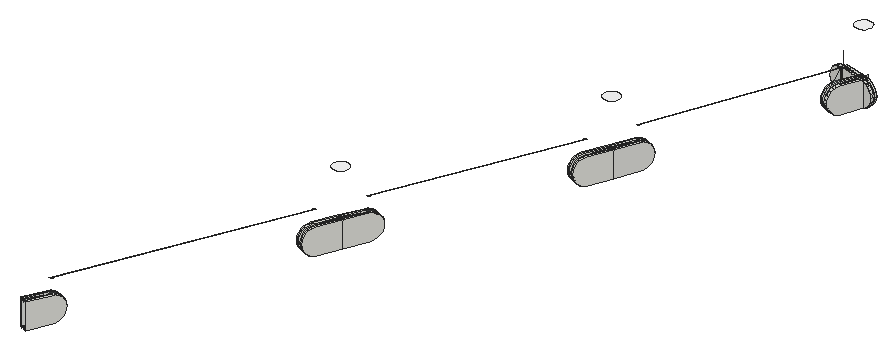
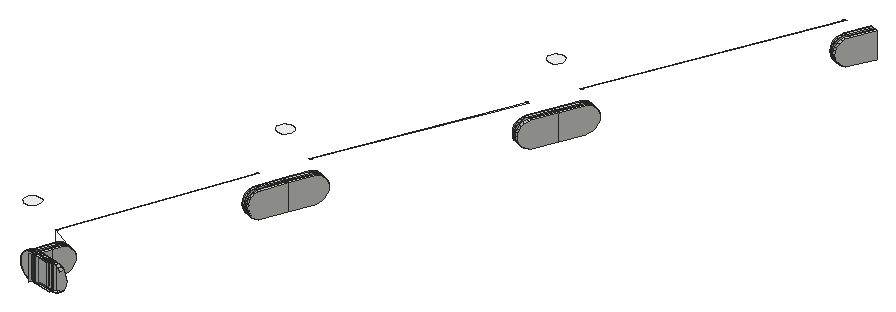
# SketchUp Ruby script. Lengths in inches.
U = 1.inch
M = Sketchup.active_model
def pt(a) = Geom::Point3d.new(a.map { |v| v * U })
def face(e, loops, mat)
  f = e.add_face(loops[0].map { |a| pt(a) })
  loops[1..].each { |l| e.add_face(l.map { |a| pt(a) }).erase! }
  f.material = f.back_material = mat if mat
  f
end
# faces: each face lists its corners as indices into pts; further lists are holes
def faces(e, pts, list, mat = nil) = list.each { |f| face(e, (f[0].is_a?(Array) ? f : [f]).map { |l| l.map { |i| pts[i] } }, mat) }
# xy, xz, yz: faces in a plane at the given z, y or x. An outline is a flat list of corners, or four numbers for a rectangle; further outlines are holes
def ring(l) = l.size == 4 ? [[l[0], l[1]], [l[2], l[1]], [l[2], l[3]], [l[0], l[3]]] : l.each_slice(2).to_a
def flat(e, list, mat, &to3) = list.each { |f| face(e, (f[0].is_a?(Array) ? f : [f]).map { |l| ring(l).map { |u, v| to3.(u, v) } }, mat) }
def xy(e, z, list, mat = nil) = flat(e, list, mat) { |x, y| [x, y, z] }
def xz(e, y, list, mat = nil) = flat(e, list, mat) { |x, z| [x, y, z] }
def yz(e, x, list, mat = nil) = flat(e, list, mat) { |y, z| [x, y, z] }
def lines(e, pts, list) = list.each { |a, b| e.add_line(pt(pts[a]), pt(pts[b])) }
# prism: a flat outline (further loops are holes) pulled along v
def prism(e, loops, v, mat = nil)
  f = face(e, loops, mat); d = Geom::Vector3d.new(v.map { |x| x * U })
  f.pushpull(f.normal.samedirection?(d) ? d.length : -d.length)
end
def box(e, o, s, mat = nil) = prism(e, [[o, [o[0] + s[0], o[1], o[2]], [o[0] + s[0], o[1] + s[1], o[2]], [o[0], o[1] + s[1], o[2]]]], [0, 0, s[2]], mat)
def at(x, y, z, deg = 0) = Geom::Transformation.translation(pt([x, y, z])) * Geom::Transformation.rotation(ORIGIN, Z_AXIS, deg.degrees)
def axes(o, x, y, z) = Geom::Transformation.new([*x, 0, *y, 0, *z, 0, *pt(o).to_a, 1])
def part(name) = M.definitions.add(name)
# library, detail: a bought-in or finely detailed component or shape, given as its bounding box
def library(name, o, s) = part(name).tap { |d| box(d.entities, o, s) }
def detail(e, o, s) = box(e.add_group.entities, o, s)
def put(e, d, t, mat = nil) = e.add_instance(d, t).tap { |i| i.material = mat if mat }
def group(e, t, mat = nil) = e.add_group.tap { |g| g.transformation = t; g.material = mat if mat }.entities
root = M.entities
M.materials.add("Glass_Safety_01").color = [204, 235, 244]
M.materials["Glass_Safety_01"].alpha = 0.1
M.materials.add("[Color_000]").color = [255, 255, 255]
xy(root,351.283,[[999.992,955.024,999.739,955.134,1000.525,956.939,1000.778,956.828],[999.558,955.212,999.306,955.322,1000.092,957.127,1000.344,957.017],[1008.551,974.677,1008.298,974.787,1008.365,974.939,1009.084,976.592,1009.337,976.482],[1008.118,974.865,1007.865,974.976,1008.651,976.78,1008.904,976.67,1008.184,975.017],[1009.337,976.482,1009.084,976.592,1009.871,978.396,1010.123,978.286],
  [1008.904,976.67,1008.651,976.78,1009.4375,978.585,1009.69,978.475],[1016.523,992.981,1016.271,993.091,1016.348,993.269,1017.057,994.896,1017.309,994.786],[1016.09,993.17,1015.837,993.28,1016.618,995.072,1016.875,994.971,1016.168,993.348],[1017.315,994.799,1017.058,994.9,1017.774,996.733,1018.031,996.633],[1016.875,994.971,1016.618,995.072,1016.621,995.078,1016.624,995.085,1016.876,994.975],
  [1016.876,994.975,1016.624,995.085,1017.334,996.905,1017.591,996.805],[1023.511,1010.674,1023.255,1010.774,1023.329,1010.964,1023.838,1012.27,1023.906,1012.255,1023.948,1012.447,1023.965,1012.524,1023.982,1012.603,1024.227,1012.508],[1023.071,1010.846,1022.815,1010.946,1023.371,1012.372,1023.644,1012.3125,1023.145,1011.036],[1023.906,1012.255,1023.838,1012.27,1023.911,1012.456,1023.948,1012.447],[1023.838,1012.27,1023.799,1012.279,1023.841,1012.471,1023.911,1012.456],
  [1023.799,1012.279,1023.644,1012.3125,1023.716,1012.498,1023.841,1012.471],[1023.644,1012.3125,1023.371,1012.372,1023.444,1012.558,1023.716,1012.498],[1023.371,1012.372,1021.983,1012.675,1022.025,1012.868,1023.251,1012.599,1023.444,1012.558],[1023.948,1012.447,1023.911,1012.456,1023.94,1012.53,1023.965,1012.524],[1023.911,1012.456,1023.841,1012.471,1023.858,1012.548,1023.94,1012.53],
  [1023.841,1012.471,1023.716,1012.498,1023.745,1012.572,1023.858,1012.548],[1023.716,1012.498,1023.444,1012.558,1023.473,1012.632,1023.745,1012.572],[1023.965,1012.524,1023.94,1012.53,1023.97,1012.608,1023.982,1012.603],[1023.94,1012.53,1023.858,1012.548,1023.745,1012.572,1023.787,1012.68,1023.53,1012.78,1023.473,1012.632,1022.042,1012.945,1022.084,1013.137,1022.095,1013.134,1022.105,1013.13,1022.106,1013.132,1023.9,1012.74,1024.007,1012.717,1023.982,1012.603,1023.97,1012.608],[1023.444,1012.558,1023.251,1012.599,1022.025,1012.868,1022.042,1012.945,1023.473,1012.632],
  [1023.745,1012.572,1023.473,1012.632,1023.53,1012.78,1023.787,1012.68],[1021.983,1012.675,1021.876,1012.699,1021.879,1012.714,1021.903,1012.702,1022.02,1012.949,1022.042,1012.945,1022.025,1012.868],[1021.903,1012.702,1021.879,1012.714,1021.935,1012.968,1022.02,1012.949]])
xy(root,351.362,[[1008.456,975.148,1008.275,975.226,1008.904,976.67,1009.084,976.592],[1009.084,976.592,1008.904,976.67,1009.533,978.114,1009.713,978.035],[1016.428,993.452,1016.247,993.531,1016.875,994.971,1016.966,994.936,1017.057,994.896],[1017.058,994.9,1016.966,994.936,1016.876,994.975,1017.447,996.438,1017.631,996.367],[1016.966,994.936,1016.875,994.971,1016.875,994.973,1016.876,994.975],
  [1023.398,1011.141,1023.214,1011.213,1023.745,1012.572,1023.858,1012.548,1023.879,1012.644,1023.97,1012.608],[1023.858,1012.548,1023.745,1012.572,1023.787,1012.68,1023.879,1012.644],[1023.745,1012.572,1023.58,1012.608,1023.622,1012.801,1023.9,1012.74,1023.879,1012.644,1023.787,1012.68],[1023.58,1012.608,1022.319,1012.884,1022.361,1013.076,1023.622,1012.801]],"Glass_Safety_01")
xy(root,353.33,[[999.739,955.134,1000.368,956.578,1000.187,956.656,999.558,955.212],[1008.456,975.148,1009.084,976.592,1008.904,976.67,1008.275,975.226],[1009.084,976.592,1009.713,978.035,1009.533,978.114,1008.904,976.67],[1016.428,993.452,1017.057,994.896,1016.966,994.936,1016.875,994.971,1016.247,993.531],[1017.058,994.9,1017.631,996.367,1017.447,996.438,1016.876,994.975,1016.966,994.936],
  [1016.966,994.936,1016.876,994.975,1016.875,994.973,1016.875,994.971],[1023.398,1011.141,1023.97,1012.608,1023.879,1012.644,1023.858,1012.548,1023.745,1012.572,1023.214,1011.213],[1023.858,1012.548,1023.879,1012.644,1023.787,1012.68,1023.745,1012.572],[1023.745,1012.572,1023.787,1012.68,1023.879,1012.644,1023.9,1012.74,1023.622,1012.801,1023.58,1012.608],[1023.58,1012.608,1023.622,1012.801,1022.361,1013.076,1022.319,1012.884]],"Glass_Safety_01")
xy(root,353.409,[[999.992,955.024,1000.778,956.828,1000.525,956.939,999.739,955.134],[999.558,955.212,1000.344,957.017,1000.092,957.127,999.306,955.322],[1008.551,974.677,1009.337,976.482,1009.084,976.592,1008.365,974.939,1008.298,974.787],[1008.118,974.865,1008.184,975.017,1008.904,976.67,1008.651,976.78,1007.865,974.976],[1009.337,976.482,1010.123,978.286,1009.871,978.396,1009.084,976.592],
  [1008.904,976.67,1009.69,978.475,1009.4375,978.585,1008.651,976.78],[1016.523,992.981,1017.309,994.786,1017.057,994.896,1016.348,993.269,1016.271,993.091],[1016.09,993.17,1016.168,993.348,1016.875,994.971,1016.618,995.072,1015.837,993.28],[1017.315,994.799,1018.031,996.633,1017.774,996.733,1017.058,994.9],[1016.875,994.971,1016.876,994.975,1016.624,995.085,1016.621,995.078,1016.618,995.072],
  [1016.876,994.975,1017.591,996.805,1017.334,996.905,1016.624,995.085],[1023.511,1010.674,1024.227,1012.508,1023.982,1012.603,1023.965,1012.524,1023.948,1012.447,1023.906,1012.255,1023.838,1012.27,1023.329,1010.964,1023.255,1010.774],[1023.071,1010.846,1023.145,1011.036,1023.644,1012.3125,1023.371,1012.372,1022.815,1010.946],[1023.906,1012.255,1023.948,1012.447,1023.911,1012.456,1023.838,1012.27],[1023.838,1012.27,1023.911,1012.456,1023.841,1012.471,1023.799,1012.279],
  [1023.799,1012.279,1023.841,1012.471,1023.716,1012.498,1023.644,1012.3125],[1023.644,1012.3125,1023.716,1012.498,1023.444,1012.558,1023.371,1012.372],[1023.371,1012.372,1023.444,1012.558,1023.251,1012.599,1022.025,1012.868,1021.983,1012.675],[1023.948,1012.447,1023.965,1012.524,1023.94,1012.53,1023.911,1012.456],[1023.911,1012.456,1023.94,1012.53,1023.858,1012.548,1023.841,1012.471],
  [1023.841,1012.471,1023.858,1012.548,1023.745,1012.572,1023.716,1012.498],[1023.716,1012.498,1023.745,1012.572,1023.473,1012.632,1023.444,1012.558],[1023.965,1012.524,1023.982,1012.603,1023.97,1012.608,1023.94,1012.53],[1023.94,1012.53,1023.97,1012.608,1023.982,1012.603,1024.007,1012.717,1023.9,1012.74,1022.106,1013.132,1022.105,1013.13,1022.095,1013.134,1022.084,1013.137,1022.042,1012.945,1023.473,1012.632,1023.53,1012.78,1023.787,1012.68,1023.745,1012.572,1023.858,1012.548],[1023.444,1012.558,1023.473,1012.632,1022.042,1012.945,1022.025,1012.868,1023.251,1012.599],
  [1023.745,1012.572,1023.787,1012.68,1023.53,1012.78,1023.473,1012.632],[1021.983,1012.675,1022.025,1012.868,1022.042,1012.945,1022.02,1012.949,1021.903,1012.702,1021.879,1012.714,1021.876,1012.699],[1021.903,1012.702,1022.02,1012.949,1021.935,1012.968,1021.879,1012.714]])
xy(root,354.511,[[1000.525,956.939,1008.184,975.017,1000.344,957.017],[1000.525,956.939,1008.365,974.939,1008.184,975.017],[1009.871,978.396,1016.168,993.348,1009.69,978.475],[1009.871,978.396,1016.348,993.269,1016.168,993.348],[1017.774,996.733,1023.145,1011.036,1017.591,996.805],
  [1017.774,996.733,1023.329,1010.964,1023.145,1011.036]],"Glass_Safety_01")
xy(root,357.267,[[1009.039,976.003,1009.2,976.036,1009.347,976.109,1009.47,976.219,1009.561,976.356,1009.613,976.512,1009.623,976.676,1009.589,976.837,1009.516,976.984,1009.407,977.107,1009.269,977.198,1009.113,977.25,1008.949,977.259,1008.788,977.226,1008.641,977.153,1008.518,977.043,1008.428,976.906,1008.376,976.75,1008.366,976.586,1008.399,976.425,1008.473,976.278,1008.582,976.155,1008.719,976.064,1008.875,976.012],[1017.011,994.307,1017.173,994.34,1017.32,994.414,1017.443,994.523,1017.533,994.66,1017.585,994.816,1017.595,994.981,1017.562,995.142,1017.488,995.289,1017.379,995.412,1017.242,995.502,1017.086,995.554,1016.921,995.564,1016.76,995.531,1016.613,995.457,1016.49,995.348,1016.4,995.211,1016.348,995.055,1016.338,994.89,1016.371,994.729,1016.445,994.582,1016.554,994.459,1016.691,994.369,1016.847,994.317],[1023.924,1012.016,1024.085,1012.049,1024.232,1012.122,1024.355,1012.231,1024.445,1012.369,1024.497,1012.525,1024.507,1012.689,1024.474,1012.85,1024.4,1012.997,1024.291,1013.12,1024.154,1013.211,1023.998,1013.262,1023.834,1013.272,1023.673,1013.239,1023.526,1013.166,1023.403,1013.056,1023.312,1012.919,1023.26,1012.763,1023.25,1012.599,1023.284,1012.438,1023.357,1012.291,1023.466,1012.168,1023.604,1012.077,1023.76,1012.025]],"[Color_000]")
p = [[1000.778,956.828,353.409],[999.992,955.024,353.409],[999.992,955.024,351.283],[1000.778,956.828,351.283],[1000.887,957.081,351.319],[1000.99,957.316,351.425],
  [1001.078,957.518,351.594],[1001.145,957.672,351.814],[1001.1875,957.77,352.071],[1001.202,957.803,352.346],[1001.1875,957.77,352.621],[1001.145,957.672,352.877],
  [1001.078,957.518,353.098],[1000.99,957.316,353.267],[1000.887,957.081,353.373],[999.739,955.134,353.409],[1000.525,956.939,353.409],[1000.525,956.939,351.283],
  [999.739,955.134,351.283],[999.739,955.134,351.362],[1000.368,956.578,351.362],[1000.368,956.578,353.33],[999.739,955.134,353.33],[999.558,955.212,351.283],
  [1000.344,957.017,351.283],[1000.344,957.017,353.409],[999.558,955.212,353.409],[999.558,955.212,353.33],[1000.187,956.656,353.33],[1000.187,956.656,351.362],
  [999.558,955.212,351.362],[999.306,955.322,353.409],[1000.092,957.127,353.409],[1000.202,957.379,353.373],[1000.304,957.614,353.267],[1000.392,957.816,353.098],
  [1000.459,957.971,352.877],[1000.502,958.069,352.621],[1000.516,958.102,352.346],[1000.502,958.069,352.071],[1000.459,957.971,351.814],[1000.392,957.816,351.594],
  [1000.304,957.614,351.425],[1000.202,957.379,351.319],[1000.092,957.127,351.283],[999.306,955.322,351.283],[1000.635,957.191,351.319],[1000.737,957.426,351.425],
  [1000.825,957.628,351.594],[1000.893,957.783,351.814],[1000.935,957.88,352.071],[1000.949,957.913,352.346],[1000.935,957.88,352.621],[1000.893,957.783,352.877],
  [1000.825,957.628,353.098],[1000.737,957.426,353.267],[1000.635,957.191,353.373],[1000.454,957.269,351.319],[1000.454,957.269,353.373],[1000.557,957.504,353.267],
  [1000.645,957.706,353.098],[1000.712,957.861,352.877],[1000.754,957.958,352.621],[1000.769,957.992,352.346],[1000.754,957.958,352.071],[1000.712,957.861,351.814],
  [1000.645,957.706,351.594],[1000.557,957.504,351.425],[1009.337,976.482,353.409],[1008.551,974.677,353.409],[1008.441,974.425,353.373],[1008.339,974.19,353.267],
  [1008.251,973.988,353.098],[1008.184,973.833,352.877],[1008.141,973.735,352.621],[1008.127,973.702,352.346],[1008.141,973.735,352.071],[1008.184,973.833,351.814],
  [1008.251,973.988,351.594],[1008.339,974.19,351.425],[1008.441,974.425,351.319],[1008.551,974.677,351.283],[1009.337,976.482,351.283],[1008.298,974.787,353.409],
  [1008.365,974.939,353.409],[1008.365,974.939,351.283],[1008.298,974.787,351.283],[1008.189,974.535,351.319],[1008.086,974.3,351.425],[1007.998,974.098,351.594],
  [1007.931,973.943,351.814],[1007.888,973.846,352.071],[1007.874,973.8125,352.346],[1007.888,973.846,352.621],[1007.931,973.943,352.877],[1007.998,974.098,353.098],
  [1008.086,974.3,353.267],[1008.189,974.535,353.373],[1008.118,974.865,351.283],[1008.184,975.017,351.283],[1008.184,975.017,353.409],[1008.118,974.865,353.409],
  [1008.008,974.613,353.373],[1007.906,974.378,353.267],[1007.818,974.176,353.098],[1007.75,974.021,352.877],[1007.708,973.924,352.621],[1007.694,973.891,352.346],
  [1007.708,973.924,352.071],[1007.75,974.021,351.814],[1007.818,974.176,351.594],[1007.906,974.378,351.425],[1008.008,974.613,351.319],[1007.865,974.976,353.409],
  [1008.651,976.78,353.409],[1008.651,976.78,351.283],[1007.865,974.976,351.283],[1007.755,974.723,351.319],[1007.653,974.488,351.425],[1007.565,974.286,351.594],
  [1007.498,974.132,351.814],[1007.455,974.034,352.071],[1007.441,974.001,352.346],[1007.455,974.034,352.621],[1007.498,974.132,352.877],[1007.565,974.286,353.098],
  [1007.653,974.488,353.267],[1007.755,974.723,353.373],[1009.084,976.592,351.283],[1009.084,976.592,353.409],[1009.084,976.592,353.33],[1008.456,975.148,353.33],
  [1008.456,975.148,351.362],[1009.084,976.592,351.362],[1008.904,976.67,353.409],[1008.904,976.67,351.283],[1008.904,976.67,351.362],[1008.275,975.226,351.362],
  [1008.275,975.226,353.33],[1008.904,976.67,353.33],[1010.123,978.286,353.409],[1010.123,978.286,351.283],[1010.233,978.539,351.319],[1010.335,978.774,351.425],
  [1010.423,978.975,351.594],[1010.491,979.13,351.814],[1010.533,979.228,352.071],[1010.548,979.261,352.346],[1010.533,979.228,352.621],[1010.491,979.13,352.877],
  [1010.423,978.975,353.098],[1010.335,978.774,353.267],[1010.233,978.539,353.373],[1009.871,978.396,353.409],[1009.871,978.396,351.283],[1009.713,978.035,351.362],
  [1009.713,978.035,353.33],[1009.69,978.475,351.283],[1009.69,978.475,353.409],[1009.533,978.114,353.33],[1009.533,978.114,351.362],[1009.4375,978.585,353.409],
  [1009.547,978.837,353.373],[1009.65,979.072,353.267],[1009.737,979.274,353.098],[1009.805,979.429,352.877],[1009.847,979.526,352.621],[1009.862,979.56,352.346],
  [1009.847,979.526,352.071],[1009.805,979.429,351.814],[1009.737,979.274,351.594],[1009.65,979.072,351.425],[1009.547,978.837,351.319],[1009.4375,978.585,351.283],
  [1009.98,978.649,351.319],[1010.083,978.884,351.425],[1010.171,979.086,351.594],[1010.238,979.24,351.814],[1010.28,979.338,352.071],[1010.295,979.371,352.346],
  [1010.28,979.338,352.621],[1010.238,979.24,352.877],[1010.171,979.086,353.098],[1010.083,978.884,353.267],[1009.98,978.649,353.373],[1009.8,978.727,351.319],
  [1009.8,978.727,353.373],[1009.902,978.962,353.267],[1009.99,979.164,353.098],[1010.058,979.319,352.877],[1010.1,979.416,352.621],[1010.114,979.45,352.346],
  [1010.1,979.416,352.071],[1010.058,979.319,351.814],[1009.99,979.164,351.594],[1009.902,978.962,351.425],[1017.309,994.786,353.409],[1016.523,992.981,353.409],
  [1016.413,992.729,353.373],[1016.311,992.494,353.267],[1016.223,992.292,353.098],[1016.156,992.137,352.877],[1016.113,992.04,352.621],[1016.099,992.007,352.346],
  [1016.113,992.04,352.071],[1016.156,992.137,351.814],[1016.223,992.292,351.594],[1016.311,992.494,351.425],[1016.413,992.729,351.319],[1016.523,992.981,351.283],
  [1017.309,994.786,351.283],[1016.271,993.091,353.409],[1016.348,993.269,353.409],[1016.348,993.269,351.283],[1016.271,993.091,351.283],[1016.161,992.839,351.319],
  [1016.058,992.604,351.425],[1015.97,992.402,351.594],[1015.903,992.247,351.814],[1015.861,992.15,352.071],[1015.846,992.117,352.346],[1015.861,992.15,352.621],
  [1015.903,992.247,352.877],[1015.97,992.402,353.098],[1016.058,992.604,353.267],[1016.161,992.839,353.373],[1016.09,993.17,351.283],[1016.168,993.348,351.283],
  [1016.875,994.971,351.283],[1016.875,994.971,351.362],[1016.875,994.971,353.33],[1016.875,994.971,353.409],[1016.168,993.348,353.409],[1016.09,993.17,353.409],
  [1015.98,992.918,353.373],[1015.878,992.683,353.267],[1015.79,992.481,353.098],[1015.723,992.326,352.877],[1015.68,992.229,352.621],[1015.666,992.195,352.346],
  [1015.68,992.229,352.071],[1015.723,992.326,351.814],[1015.79,992.481,351.594],[1015.878,992.683,351.425],[1015.98,992.918,351.319],[1015.837,993.28,353.409],
  [1016.618,995.072,353.409],[1016.618,995.072,351.283],[1015.837,993.28,351.283],[1015.728,993.028,351.319],[1015.625,992.793,351.425],[1015.537,992.591,351.594],
  [1015.47,992.436,351.814],[1015.427,992.339,352.071],[1015.413,992.306,352.346],[1015.427,992.339,352.621],[1015.47,992.436,352.877],[1015.537,992.591,353.098],
  [1015.625,992.793,353.267],[1015.728,993.028,353.373],[1017.057,994.896,351.283],[1017.057,994.896,353.409],[1017.057,994.896,353.33],[1016.428,993.452,353.33],
  [1016.428,993.452,351.362],[1017.057,994.896,351.362],[1017.058,994.9,351.362],[1017.058,994.9,351.283],[1017.315,994.799,351.283],[1017.315,994.799,353.409],
  [1017.058,994.9,353.409],[1017.058,994.9,353.33],[1018.031,996.633,353.409],[1018.031,996.633,351.283],[1018.131,996.89,351.319],[1018.224,997.128,351.425],
  [1018.304,997.333,351.594],[1018.365,997.491,351.814],[1018.404,997.59,352.071],[1018.417,997.623,352.346],[1018.404,997.59,352.621],[1018.365,997.491,352.877],
  [1018.304,997.333,353.098],[1018.224,997.128,353.267],[1018.131,996.89,353.373],[1017.774,996.733,353.409],[1017.774,996.733,351.283],[1017.631,996.367,351.362],
  [1017.631,996.367,353.33],[1016.876,994.975,351.362],[1016.876,994.975,351.283],[1016.624,995.085,351.283],[1016.624,995.085,353.409],[1016.876,994.975,353.409],
  [1016.876,994.975,353.33],[1017.591,996.805,351.283],[1017.691,997.061,351.319],[1017.784,997.3,351.425],[1017.864,997.505,351.594],[1017.925,997.663,351.814],
  [1017.964,997.762,352.071],[1017.977,997.795,352.346],[1017.964,997.762,352.621],[1017.925,997.663,352.877],[1017.864,997.505,353.098],[1017.784,997.3,353.267],
  [1017.691,997.061,353.373],[1017.591,996.805,353.409],[1016.621,995.078,351.283],[1016.621,995.078,353.409],[1017.334,996.905,353.409],[1017.434,997.162,353.373],
  [1017.527,997.4,353.267],[1017.607,997.605,353.098],[1017.669,997.763,352.877],[1017.707,997.862,352.621],[1017.72,997.895,352.346],[1017.707,997.862,352.071],
  [1017.669,997.763,351.814],[1017.607,997.605,351.594],[1017.527,997.4,351.425],[1017.434,997.162,351.319],[1017.334,996.905,351.283],[1017.874,996.99,351.319],
  [1017.967,997.229,351.425],[1018.047,997.434,351.594],[1018.109,997.591,351.814],[1018.147,997.69,352.071],[1018.16,997.724,352.346],[1018.147,997.69,352.621],
  [1018.109,997.591,352.877],[1018.047,997.434,353.098],[1017.967,997.229,353.267],[1017.874,996.99,353.373],[1024.227,1012.508,353.409],[1023.511,1010.674,353.409],
  [1023.411,1010.418,353.373],[1023.318,1010.179,353.267],[1023.238,1009.974,353.098],[1023.177,1009.817,352.877],[1023.138,1009.718,352.621],[1023.125,1009.684,352.346],
  [1023.138,1009.718,352.071],[1023.177,1009.817,351.814],[1023.238,1009.974,351.594],[1023.318,1010.179,351.425],[1023.411,1010.418,351.319],[1023.511,1010.674,351.283],
  [1024.227,1012.508,351.283],[1023.329,1010.964,353.409],[1023.329,1010.964,351.283],[1023.255,1010.774,351.283],[1023.155,1010.518,351.319],[1023.061,1010.279,351.425],
  [1022.981,1010.074,351.594],[1022.92,1009.917,351.814],[1022.881,1009.818,352.071],[1022.868,1009.784,352.346],[1022.881,1009.818,352.621],[1022.908,1009.886,352.798],
  [1022.981,1010.074,353.098],[1022.982,1010.075,353.098],[1023.061,1010.279,353.267],[1023.155,1010.518,353.373],[1023.255,1010.774,353.409],[1023.071,1010.846,351.283],
  [1023.145,1011.036,351.283],[1023.145,1011.036,353.409],[1023.071,1010.846,353.409],[1022.971,1010.59,353.373],[1022.878,1010.351,353.267],[1022.798,1010.146,353.098],
  [1022.737,1009.988,352.877],[1022.698,1009.889,352.621],[1022.685,1009.856,352.346],[1022.698,1009.889,352.071],[1022.737,1009.988,351.814],[1022.798,1010.146,351.594],
  [1022.878,1010.351,351.425],[1022.971,1010.59,351.319],[1023.473,1012.632,353.409],[1023.53,1012.78,353.409],[1023.53,1012.78,351.283],[1023.473,1012.632,351.283],
  [1023.444,1012.558,351.283],[1023.371,1012.372,351.283],[1022.815,1010.946,351.283],[1022.715,1010.69,351.319],[1022.621,1010.451,351.425],[1022.541,1010.246,351.594],
  [1022.48,1010.089,351.814],[1022.441,1009.99,352.071],[1022.428,1009.956,352.346],[1022.441,1009.99,352.621],[1022.48,1010.089,352.877],[1022.541,1010.246,353.098],
  [1022.621,1010.451,353.267],[1022.715,1010.69,353.373],[1022.815,1010.946,353.409],[1023.371,1012.372,353.409],[1023.444,1012.558,353.409],[1023.644,1012.3125,353.409],
  [1023.644,1012.3125,351.283],[1023.716,1012.498,351.283],[1023.745,1012.572,351.283],[1023.787,1012.68,351.283],[1023.787,1012.68,351.362],[1023.745,1012.572,351.362],
  [1023.214,1011.213,351.362],[1023.214,1011.213,353.33],[1023.745,1012.572,353.33],[1023.787,1012.68,353.33],[1023.787,1012.68,353.409],[1023.745,1012.572,353.409],
  [1023.716,1012.498,353.409],[1023.838,1012.27,351.283],[1023.838,1012.27,353.409],[1023.911,1012.456,353.409],[1023.94,1012.53,353.409],[1023.97,1012.608,353.409],
  [1023.97,1012.608,353.33],[1023.398,1011.141,353.33],[1023.398,1011.141,351.362],[1023.97,1012.608,351.362],[1023.97,1012.608,351.283],[1023.94,1012.53,351.283],
  [1023.911,1012.456,351.283],[1023.799,1012.279,353.409],[1023.799,1012.279,351.283],[1023.906,1012.255,351.283],[1024.175,1012.196,351.319],[1024.425,1012.142,351.425],
  [1024.641,1012.095,351.594],[1024.806,1012.059,351.814],[1024.909,1012.036,352.071],[1024.945,1012.028,352.346],[1024.909,1012.036,352.621],[1024.806,1012.059,352.877],
  [1024.641,1012.095,353.098],[1024.425,1012.142,353.267],[1024.175,1012.196,353.373],[1023.906,1012.255,353.409],[1024.217,1012.389,351.319],[1024.467,1012.334,351.425],
  [1023.251,1012.599,353.409],[1022.025,1012.868,353.409],[1022.025,1012.868,351.283],[1023.251,1012.599,351.283],[1023.841,1012.471,351.283],[1023.948,1012.447,351.283],
  [1024.683,1012.287,351.594],[1024.848,1012.251,351.814],[1024.951,1012.228,352.071],[1024.987,1012.22,352.346],[1024.951,1012.228,352.621],[1024.848,1012.251,352.877],
  [1024.683,1012.287,353.098],[1024.467,1012.334,353.267],[1024.217,1012.389,353.373],[1023.948,1012.447,353.409],[1023.841,1012.471,353.409],[1021.983,1012.675,353.409],
  [1021.983,1012.675,351.283],[1023.858,1012.548,351.283],[1023.858,1012.548,351.362],[1023.858,1012.548,353.33],[1023.858,1012.548,353.409],[1023.965,1012.524,353.409],
  [1024.234,1012.466,353.373],[1024.484,1012.411,353.267],[1024.699,1012.364,353.098],[1024.864,1012.328,352.877],[1024.968,1012.305,352.621],[1025.003,1012.297,352.346],
  [1024.968,1012.305,352.071],[1024.864,1012.328,351.814],[1024.699,1012.364,351.594],[1024.484,1012.411,351.425],[1024.234,1012.466,351.319],[1023.965,1012.524,351.283],
  [1024.276,1012.658,351.319],[1024.526,1012.603,351.425],[1023.58,1012.608,353.33],[1023.58,1012.608,351.362],[1022.042,1012.945,351.283],[1022.042,1012.945,351.362],
  [1022.319,1012.884,351.362],[1022.319,1012.884,353.33],[1022.042,1012.945,353.33],[1022.042,1012.945,353.409],[1024.007,1012.717,351.283],[1023.9,1012.74,351.283],
  [1023.9,1012.74,351.362],[1023.9,1012.74,353.33],[1023.9,1012.74,353.409],[1024.007,1012.717,353.409],[1024.276,1012.658,353.373],[1024.526,1012.603,353.267],
  [1024.741,1012.556,353.098],[1024.906,1012.52,352.877],[1025.01,1012.497,352.621],[1025.046,1012.49,352.346],[1025.01,1012.497,352.071],[1024.906,1012.52,351.814],
  [1024.741,1012.556,351.594],[1023.982,1012.603,353.409],[1023.982,1012.603,351.283],[1021.876,1012.699,351.283],[1021.876,1012.699,353.409],[1021.607,1012.757,353.373],
  [1021.357,1012.812,353.267],[1021.141,1012.859,353.098],[1020.976,1012.895,352.877],[1020.873,1012.918,352.621],[1020.837,1012.926,352.346],[1020.873,1012.918,352.071],
  [1020.976,1012.895,351.814],[1021.141,1012.859,351.594],[1021.357,1012.812,351.425],[1021.607,1012.757,351.319],[1021.666,1013.027,351.319],[1021.928,1012.969,351.284],
  [1021.935,1012.968,351.283],[1021.879,1012.714,351.283],[1022.021,1012.952,351.283],[1022.021,1012.952,351.362],[1022.021,1012.952,353.33],[1022.021,1012.952,353.409],
  [1022.02,1012.949,353.409],[1021.903,1012.702,353.409],[1021.903,1012.702,351.283],[1022.02,1012.949,351.283],[1023.959,1013.009,351.283],[1023.959,1013.009,353.409],
  [1021.415,1013.081,351.425],[1021.935,1012.968,353.409],[1021.928,1012.969,353.408],[1016.247,993.531,353.33],[1016.247,993.531,351.362],[1016.966,994.936,351.362],
  [1016.966,994.936,353.33],[1016.875,994.973,353.33],[1016.875,994.973,351.362],[1017.447,996.438,351.362],[1017.447,996.438,353.33],[1023.879,1012.644,351.362],
  [1023.879,1012.644,353.33],[1023.622,1012.801,351.362],[1023.622,1012.801,353.33],[1021.2,1013.128,351.594],[1022.361,1013.076,353.33],[1022.361,1013.076,351.362],
  [1022.92,1009.917,352.877],[1023.329,1010.964,354.511],[1021.415,1013.081,353.267],[1021.2,1013.128,353.098],[1021.666,1013.027,353.373],[1021.879,1012.714,353.409],
  [1021.928,1012.969,354.511],[1021.935,1012.968,354.511]]
faces(root,p,[[0,1,2,3,4,5,6,7,8,9,10,11,12,13,14],[15,16,17,18,19,20,21,22],[23,24,25,26,27,28,29,30],[31,32,33,34,35,36,37,38,39,40,41,42,43,44,45],[17,46,4,3],[57,24,44,43],[46,47,5,4],[67,57,43,42],
  [68,69,70,71,72,73,74,75,76,77,78,79,80,81,82],[83,84,85,86,87,88,89,90,91,92,93,94,95,96,97],[98,99,100,101,102,103,104,105,106,107,108,109,110,111,112],[113,114,115,116,117,118,119,120,121,122,123,124,125,126,127],[88,87,80,79],[112,111,118,117],[87,86,81,80],[98,112,117,116],
  [128,85,84,129,130,131,132,133],[134,100,99,135,136,137,138,139],[128,133,130,129,68,82],[140,68,82,141,142,143,144,145,146,147,148,149,150,151,152],[129,153,154,128,133,155,156,130],[136,135,115,114,134,139],[135,157,158,134,139,159,160,136],[114,161,162,163,164,165,166,167,168,169,170,171,172,173,115],
  [154,174,142,141],[185,157,173,172],[174,175,143,142],[195,185,172,171],[196,197,198,199,200,201,202,203,204,205,206,207,208,209,210],[211,212,213,214,215,216,217,218,219,220,221,222,223,224,225],[226,227,228,229,230,231,232,233,234,235,236,237,238,239,240,241,242,243,244],[245,246,247,248,249,250,251,252,253,254,255,256,257,258,259],
  [216,215,208,207],[244,243,250,249],[215,214,209,208],[226,244,249,248],[260,213,212,261,262,263,264,265],[260,265,262,261,196,210],[266,267,268,269,270,271],[272,269,268,273,274,275,276,277,278,279,280,281,282,283,284],
  [270,285,286,267,266,287,288,271],[228,229,230,231,246,247],[289,290,291,292,293,294],[293,231,230,229,228,290,289,294],[293,231,230,229,228,290,295,296,297,298,299,300,301,302,303,304,305,306,307],[308,247,246,309,292,291],[246,309,292,310,311,312,313,314,315,316,317,318,319,320,321,322,291,308,247],[286,323,274,273],
  [296,295,322,321],[323,324,275,274],[297,296,321,320],[334,335,336,337,338,339,340,341,342,343,344,345,346,347,348],[365,366,367,368,369,370,371,372,373,374,375,376,377,378,379],[380,381,382,383,384,385,386,387,388,389,390,391,392,393,394,395,396,397,398,399,400],[353,352,346,345],[379,378,388,387],
  [352,351,347,346],[365,379,387,386],[401,367,366,402,403,404,405,406,407,408,409,410,411,412,413,414],[415,350,349,416,417,418,419,420,421,422,423,424,425,426],[416,427,428,415,429,430,431,432,433,434,435,436,437,438,439,440,441],[430,442,443,431],[444,445,446,447,384,403,448,426,449,442,443,450,451,452,453,454,455,456,457,458,459,417,460,414,400],[429,449,442,430],
  [402,428,427,401,399,461,462,385],[463,464,465,466,460,427,428,448],[425,463,464,465,466,418,467,468,469,470,471,472,473,474,475,476,477,478,479],[477,443,442,478],[478,442,449,479],[480,481,477,478],[413,466,465,410,482,483,407,464,463,404,383,484,485,486,487,488,489,380],[490,491,492,493,494,495,496,497,498,499,500,501,502,503,504,481,480],
  [424,423,420,419,505,334,348,506],[490,480,478,479,506],[507,462,461,508,509,510,511,512,513,514,515,516,517,518,519],[520,521,522,523,507,519],[524,525,526,527,528,529,530,531],[445,461,462,446],[406,405,382,381,412,411],[492,491,532,533,494,493],
  [534,520,519,518],[531,522,535,528,489,488,485,484],[484,485,488,489,445,446],[47,48,6,5],[66,67,42,41],[89,88,79,78],[111,110,119,118],[175,176,144,143],
  [194,195,171,170],[217,216,207,206],[243,242,251,250],[324,325,276,275],[298,297,320,319],[354,353,345,344],[378,377,389,388],[431,443,450,432],
  [476,450,443,477],[481,504,476,477],[549,534,518,517],[485,488,487,486],[48,49,7,6],[65,66,41,40],[90,89,78,77],[110,109,120,119],
  [176,177,145,144],[193,194,170,169],[218,217,206,205],[242,241,252,251],[325,326,277,276],[299,298,319,318],[355,354,344,343],[377,376,390,389],
  [432,450,451,433],[475,451,450,476],[504,503,475,476],[49,50,8,7],[64,65,40,39],[91,90,77,76],[109,108,121,120],[177,178,146,145],
  [192,193,169,168],[219,218,205,204],[241,240,253,252],[326,327,278,277],[300,299,318,317],[356,355,343,342],[376,375,391,390],[433,451,452,434],
  [474,452,451,475],[503,502,474,475],[50,51,9,8],[63,64,39,38],[92,91,76,75],[108,107,122,121],[178,179,147,146],[191,192,168,167],
  [220,219,204,203],[240,239,254,253],[327,328,279,278],[301,300,317,316],[357,356,342,341],[375,374,392,391],[434,452,453,435],[473,453,452,474],
  [502,501,473,474],[51,52,10,9],[62,63,38,37],[93,92,75,74],[107,106,123,122],[179,180,148,147],[190,191,167,166],[221,220,203,202],
  [239,238,255,254],[328,329,280,279],[302,301,316,315],[358,357,341,340],[374,373,393,392],[435,453,454,436],[472,454,453,473],[501,500,472,473],
  [52,53,11,10],[61,62,37,36],[94,93,74,73],[106,105,124,123],[180,181,149,148],[189,190,166,165],[222,221,202,201],[238,237,256,255],
  [329,330,281,280],[303,302,315,314],[552,359,358,340,339],[373,372,394,393],[436,454,455,437],[471,455,454,472],[500,499,471,472],[359,552,360],
  [53,54,12,11],[60,61,36,35],[95,94,73,72],[105,104,125,124],[181,182,150,149],[188,189,165,164],[223,222,201,200],[237,236,257,256],
  [330,331,282,281],[304,303,314,313],[360,552,339,338],[372,371,395,394],[437,455,456,438],[470,456,455,471],[499,498,470,471],[54,55,13,12],
  [59,60,35,34],[96,95,72,71],[104,103,126,125],[182,183,151,150],[187,188,164,163],[224,223,200,199],[236,235,258,257],[331,332,283,282],
  [305,304,313,312],[362,361,360,338,337],[371,370,396,395],[438,456,457,439],[469,457,456,470],[498,497,469,470],[554,555,511,510],[55,56,14,13],
  [58,59,34,33],[97,96,71,70],[103,102,127,126],[183,184,152,151],[186,187,163,162],[225,224,199,198],[235,234,259,258],[332,333,284,283],
  [306,305,312,311],[363,362,337,336],[370,369,397,396],[439,457,458,440],[468,458,457,469],[497,496,468,469],[556,554,510,509],[56,16,0,14],
  [25,58,33,32],[83,97,70,69],[102,101,113,127],[184,153,140,152],[158,186,162,161],[211,225,198,197],[234,233,245,259],[333,285,272,284],
  [307,306,311,310],[364,363,336,335],[369,368,398,397],[458,440,441,459],[467,505,495,496,468,458,459],[535,536,556,509,508,557]])
faces(root,p,[[16,17,46,47,48,49,50,51,52,53,54,55,56],[24,25,58,59,60,61,62,63,64,65,66,67,57],[153,154,174,175,176,177,178,179,180,181,182,183,184],[157,158,186,187,188,189,190,191,192,193,194,195,185],[285,286,323,324,325,326,327,328,329,330,331,332,333],[295,307,306,305,304,303,302,301,300,299,298,297,296],[349,350,351,352,353,354,355,356,357,358,359,360,361,362,363,364],[522,535,536,521],
  [28,27,30,29],[21,20,29,28],[138,137,132,131],[131,130,133,132],[139,138,137,136],[139,130,133,136],[130,156,155,133],[159,139,136,160],
  [156,155,160,159],[537,538,264,263],[537,230,229,538],[263,262,265,264],[539,540,230,229],[294,540,539,289],[265,539,540,262],[540,539,266,271],
  [271,288,287,266],[541,294,289,542,229,230],[543,289,294,544],[287,543,544,288],[409,408,422,421],[421,420,423,422],[411,410,409,408,407,406],[482,410,465,464,407,483],
  [545,546,465,464],[482,487,486,483],[482,483,547,548],[411,546,545,406],[423,545,546,420],[546,545,492,493],[492,547,548,493],[550,548,547,551],
  [551,486,487,550],[553,361,362,363,364,349],[558,536,535,559]],"Glass_Safety_01")
